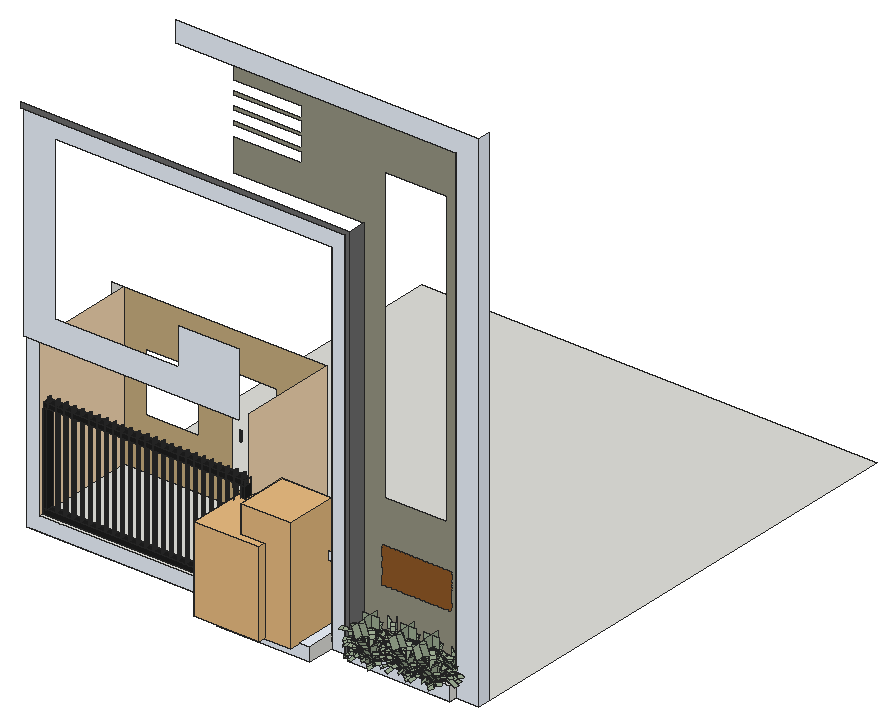
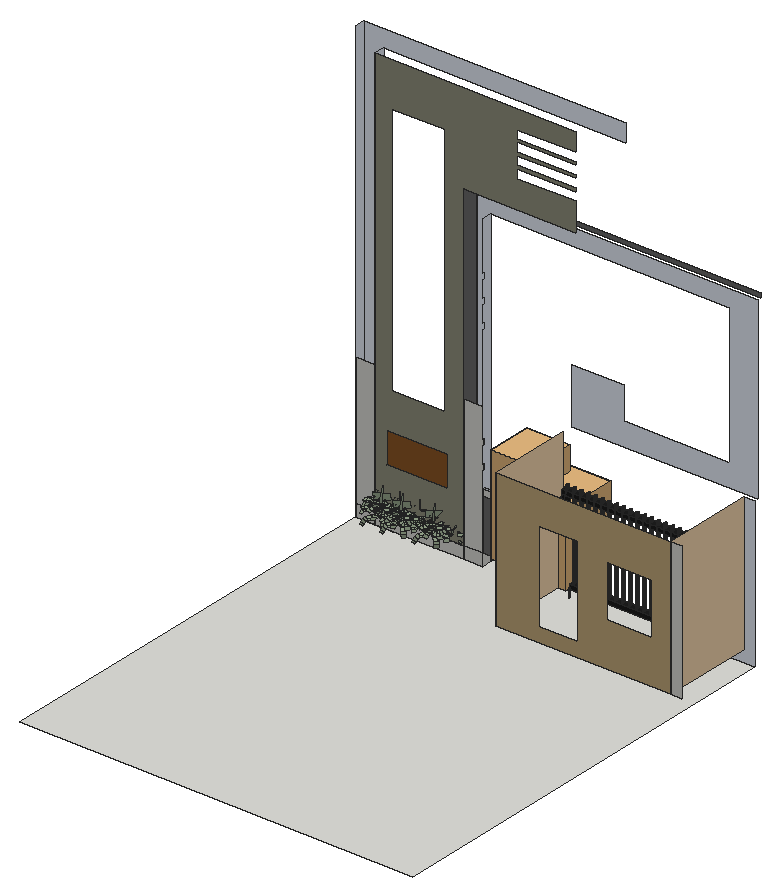
# SketchUp Ruby script. Lengths in inches.
U = 1.inch
M = Sketchup.active_model
def pt(a) = Geom::Point3d.new(a.map { |v| v * U })
def face(e, loops, mat)
  f = e.add_face(loops[0].map { |a| pt(a) })
  loops[1..].each { |l| e.add_face(l.map { |a| pt(a) }).erase! }
  f.material = f.back_material = mat if mat
  f
end
# faces: each face lists its corners as indices into pts; further lists are holes
def faces(e, pts, list, mat = nil) = list.each { |f| face(e, (f[0].is_a?(Array) ? f : [f]).map { |l| l.map { |i| pts[i] } }, mat) }
# xy, xz, yz: faces in a plane at the given z, y or x. An outline is a flat list of corners, or four numbers for a rectangle; further outlines are holes
def ring(l) = l.size == 4 ? [[l[0], l[1]], [l[2], l[1]], [l[2], l[3]], [l[0], l[3]]] : l.each_slice(2).to_a
def flat(e, list, mat, &to3) = list.each { |f| face(e, (f[0].is_a?(Array) ? f : [f]).map { |l| ring(l).map { |u, v| to3.(u, v) } }, mat) }
def xy(e, z, list, mat = nil) = flat(e, list, mat) { |x, y| [x, y, z] }
def xz(e, y, list, mat = nil) = flat(e, list, mat) { |x, z| [x, y, z] }
def yz(e, x, list, mat = nil) = flat(e, list, mat) { |y, z| [x, y, z] }
def lines(e, pts, list) = list.each { |a, b| e.add_line(pt(pts[a]), pt(pts[b])) }
# prism: a flat outline (further loops are holes) pulled along v
def prism(e, loops, v, mat = nil)
  f = face(e, loops, mat); d = Geom::Vector3d.new(v.map { |x| x * U })
  f.pushpull(f.normal.samedirection?(d) ? d.length : -d.length)
end
def box(e, o, s, mat = nil) = prism(e, [[o, [o[0] + s[0], o[1], o[2]], [o[0] + s[0], o[1] + s[1], o[2]], [o[0], o[1] + s[1], o[2]]]], [0, 0, s[2]], mat)
def at(x, y, z, deg = 0) = Geom::Transformation.translation(pt([x, y, z])) * Geom::Transformation.rotation(ORIGIN, Z_AXIS, deg.degrees)
def axes(o, x, y, z) = Geom::Transformation.new([*x, 0, *y, 0, *z, 0, *pt(o).to_a, 1])
def part(name) = M.definitions.add(name)
# library, detail: a bought-in or finely detailed component or shape, given as its bounding box
def library(name, o, s) = part(name).tap { |d| box(d.entities, o, s) }
def detail(e, o, s) = box(e.add_group.entities, o, s)
def put(e, d, t, mat = nil) = e.add_instance(d, t).tap { |i| i.material = mat if mat }
def group(e, t, mat = nil) = e.add_group.tap { |g| g.transformation = t; g.material = mat if mat }.entities
root = M.entities
M.materials.add("Generic").color = [111, 111, 111]
M.materials.add("Generic\#2").color = [253, 222, 182]
M.materials.add("Generic\#3").color = [151, 150, 132]
M.materials.add("Generic\#4").color = [238, 245, 255]
M.materials.add("Material \#1").color = [140, 140, 140]
M.materials.add("[Color M08]").color = [30, 30, 30]
M.materials.add("[Roofing Slate Tan]").color = [200, 175, 128]
M.materials.add("[Wood Floor Parquet]").color = [145, 89, 39]
M.materials.add("hymenocallis littoralis").color = [156, 172, 146]
c1 = library("Plant+2 (1)",[-9.13,-9.52,0],[51.76,51.77,66.88])
c2 = library("Plant",[-27.84,-31.84,-1.26],[68.28,70.82,154.38])
c3 = part("Group\#856")
xy(c3.entities,7.38,[[0,0,5.5,15.91]],"hymenocallis littoralis")
p = [[5.5,28.78,0],[5.5,26.79,3.44],[0,26.79,3.44],[0,28.78,0],[0,23.75,6],[5.5,23.75,6],
  [0,15.91,7.38],[5.5,15.91,7.38]]
faces(c3.entities,p,[[0,1,2,3],[4,2,1,5],[6,4,5,7]],"hymenocallis littoralis")
c4 = part("Group\#854")
xy(c4.entities,7.38,[[0,0,5.5,15.91],[0,15.91,5.5,23.87]],"hymenocallis littoralis")
p = [[5.5,31.07,4.3],[5.5,27.74,6.47],[0,27.74,6.47],[0,31.07,4.3],[0,23.87,7.38],[5.5,23.87,7.38]]
faces(c4.entities,p,[[0,1,2,3],[4,2,1,5]],"hymenocallis littoralis")
c5 = part("Group\#857")
xy(c5.entities,7.38,[[0,0,5.6,15.91]],"hymenocallis littoralis")
p = [[5.6,28.78,0],[5.6,26.79,3.44],[0,26.79,3.44],[0,28.78,0],[0,23.75,6],[5.6,23.75,6],
  [0,15.91,7.38],[5.6,15.91,7.38]]
faces(c5.entities,p,[[0,1,2,3],[4,2,1,5],[6,4,5,7]],"hymenocallis littoralis")
c6 = part("Group\#855")
put(c6.entities,c4,axes([6.09,8.57,-0.52],[0.446,0.85617,0.26089],[-0.18444,-0.19731,0.96283],[0.87582,-0.47754,0.0699]))
put(c6.entities,c4,axes([6.29,7.28,-1.71],[0.37058,0.92707,-0.05667],[-0.32382,0.19004,0.99128],[0.87712,-0.32925,0.34964]))
put(c6.entities,c4,axes([11.04,16.14,-0.7],[1,0,0],[0,0.16628,1.02662],[0,-1.18456,0.19186]))
c7 = part("Group\#860")
put(c7.entities,c3,axes([24.57,32.05,-1.76],[0.9552,-0.22102,-0.19681],[0.4036,0.95545,0.88585],[-0.00568,-0.67859,0.7345]))
put(c7.entities,c3,axes([23.95,29.24,-2.4],[0,1,0],[-0.76041,0,0.64945],[0.64945,0,0.76041]))
put(c7.entities,c3,axes([24.22,24.72,-0.48],[-0.70711,0.70711,0],[-0.32757,-0.32757,0.80237],[0.61237,0.61237,0.5]))
put(c7.entities,c4,axes([20.66,37.22,-0.63],[1.12361,0.03262,0.39091],[-0.43499,0.29739,0.78777],[0.09852,-1.27434,0.37535]))
put(c7.entities,c3,axes([28.75,24.45,-2.4],[-1,0,0],[0,-0.76041,0.64945],[0,0.64945,0.76041]))
put(c7.entities,c5,axes([30.4,30.98,-3.7],[0.65676,-0.72002,0.22414],[0.55667,0.66341,0.5],[-0.50871,-0.20361,0.83652]))
put(c7.entities,c5,axes([32.41,29.61,-3.7],[0.04029,-0.97372,0.22414],[0.85287,0.15038,0.5],[-0.52057,0.17102,0.83652]))
put(c7.entities,c3,axes([31.89,25.85,-1.76],[-0.92056,0.33739,-0.19681],[-0.5186,-0.89824,0.88585],[0.08952,0.67268,0.7345]))
put(c7.entities,c3,axes([25.55,34.78,-0.48],[0.86603,0.5,0],[-0.25,0.43301,0.86603],[0.43301,-0.75,0.5]))
put(c7.entities,c5,axes([20.4,16.9375,-8.07],[-0.70711,0.70711,0],[-0.35754,-0.35754,0.65422],[1.3987,1.3987,1.52882]))
put(c7.entities,c3,axes([32.86,34.14,-0.48],[0.76604,-0.64279,0],[0.32139,0.38302,0.86603],[-0.55667,-0.66341,0.5]))
put(c7.entities,c3,axes([27.15,34.7,-0.1],[0.82472,-0.17528,-0.53769],[0.53769,0.53769,0.64945],[0.17528,-0.82472,0.53769]))
put(c7.entities,c3,axes([33.58,28.77,-2.4],[0,-1,0],[0.76041,0,0.64945],[-0.64945,0,0.76041]))
put(c7.entities,c3,axes([26.43,23.87,-2.81],[-0.75126,0.04415,0.65853],[0.53769,-0.53769,0.64945],[0.38276,0.84199,0.3802]))
put(c7.entities,c3,axes([28.78,23.98,-2.4],[-1,0,0],[0,-0.76041,0.64945],[0,0.64945,0.76041]))
put(c7.entities,c3,axes([25.39,25.38,-2.4],[-0.70711,0.70711,0],[-0.53769,-0.53769,0.64945],[0.45923,0.45923,0.76041]))
put(c7.entities,c3,axes([27.32,21.63,-0.1],[-0.45923,0.70711,-0.53769],[-0.76041,0,0.64945],[0.45923,0.70711,0.53769]))
put(c7.entities,c3,axes([25.17,27.625,-1.76],[0.56416,0.80187,-0.19681],[-0.66673,0.66673,0.80532],[0.62659,-0.26057,0.7345]))
put(c7.entities,c5,axes([27.59,27.04,-3.96],[-0.8993,-0.06127,0.43301],[0.2962,-0.8138,0.5],[0.32175,0.57791,0.75]))
put(c7.entities,c5,axes([26.98,24.5,-3.18],[-0.5,0.86603,0],[-0.75,-0.43301,0.5],[0.43301,0.25,0.86603]))
put(c7.entities,c5,axes([24.55,27.74,-3.7],[0.29517,0.92878,0.22414],[-0.85287,0.15038,0.5],[0.43068,-0.33875,0.83652]))
put(c7.entities,c5,axes([24.26,29.8,-3.18],[0.76604,0.64279,0],[-0.47317,0.5639,0.425],[0.32139,-0.38302,0.86603]))
put(c7.entities,c5,axes([25.98,32.46,-3.18],[1,0,0],[0,0.86603,0.5],[0,-0.5,0.86603]))
put(c7.entities,c3,axes([28.78,33.57,-2.4],[1,0,0],[0,0.76041,0.64945],[0,-0.64945,0.76041]))
put(c7.entities,c6,at(14.99,21.38,2.5))
put(c7.entities,c4,axes([34.63,26.34,-1.46],[-0.70089,-0.70877,0.07994],[0.4756,-0.38088,0.79293],[-0.53156,0.59378,0.60405]))
put(c7.entities,c4,axes([28.14,16.92,1.8125],[-1.19719,0.6912,0],[-0.09607,-0.16641,0.94244],[0.68444,1.18549,0.17613]))
put(c7.entities,c4,axes([31.5625,35.84,0.97],[0.66765,-1.1564,0.35779],[0.04445,0.30732,0.91033],[-1.20828,-0.64496,0.17012]))
put(c7.entities,c4,axes([38.94,22.51,0.89],[-0.97932,-0.67164,-0.05202],[0.27787,-0.41401,0.90999],[-0.85985,0.93577,0.32097]))
put(c7.entities,c4,axes([38.44,21.09,1.98],[-1.02864,-0.54856,0.2395],[0.33481,0.06999,0.88388],[-0.77261,1.08328,0.06417]))
put(c7.entities,c5,axes([35.02,30.51,-1.3],[-0.17365,-0.98481,0],[0.60224,-0.10619,0.79122],[-0.7792,0.13739,0.61153]))
put(c7.entities,c5,axes([29.41,22.33,-1.3],[-0.93969,0.34202,0],[-0.20915,-0.57465,0.79122],[0.27061,0.74351,0.61153]))
put(c7.entities,c4,axes([19.64,36,-1.62],[1.18194,0.09546,0.08234],[-0.14377,0.68823,0.76313],[0.21457,-1.1326,0.62386]))
put(c7.entities,c5,axes([24.25,24.14,-1.3],[-0.34202,0.93969,0],[-0.57465,-0.20915,0.79122],[0.74351,0.27061,0.61153]))
put(c7.entities,c5,axes([25.98,34.61,-1.3],[1,0,0],[0,0.61153,0.79122],[0,-0.79122,0.61153]))
put(c7.entities,c5,axes([31.16,34.41,-1.64],[0.56518,-0.80224,-0.19234],[0.73413,0.34233,0.72935],[-0.47639,-0.50772,0.71782]))
put(c7.entities,c5,axes([40.52,26.84,-5.82],[-0.42262,-0.90631,0],[0.48019,-0.22391,0.68552],[-1.43418,0.66877,1.22305]))
put(c7.entities,c3,axes([29.86,38.42,-1.01],[0.89064,-0.37013,0.26413],[-0.03924,0.63286,1.01918],[-0.45353,-0.76487,0.45748]))
put(c7.entities,c3,axes([29.34,22.4,-0.48],[-0.99619,-0.08716,0],[0.04358,-0.4981,0.86603],[-0.07548,0.86273,0.5]))
c8 = part("Group\#858")
xz(c8.entities,10.07,[[9.07,0,10.07,31.01],[0,31.01,0,45.12,20.13,45.12,20.13,31.01,10.07,31.01,10.07,32.58,9.07,32.58,9.07,31.01]],"hymenocallis littoralis")
yz(c8.entities,10.07,[[0,31.01,20.13,45.12]],"hymenocallis littoralis")
p = [[9.57,9.2,0],[10.07,10.07,0],[10.07,10.07,31.01],[10.07,10.07,32.58],[9.57,9.2,32.58]]
faces(c8.entities,p,[[0,1,2,3,4]],"hymenocallis littoralis")
c9 = part("cây lá nắng")
put(c9.entities,c7,axes([49.26,-2.75,0],[0.63109,0.63109,0],[-0.63109,0.63109,0],[0,0,0.935]))
g1 = group(c9.entities,at(26.6,-8.68,0))
put(g1,c3,axes([-4.72,35.73,-1.65],[0.74231,0.46334,-0.18402],[-0.34827,0.85768,0.82827],[0.42467,-0.43184,0.68675]))
put(g1,c3,axes([-3.34,33.57,-2.24],[-0.63109,0.63109,0],[-0.47989,-0.47989,0.60723],[0.40986,0.40986,0.71098]))
put(g1,c3,axes([-0.3125,30.89,-0.45],[-0.8925,0,0],[0,-0.41345,0.75022],[0,0.77293,0.4675]))
put(g1,c4,axes([-10.79,39.66,-0.59],[0.68852,0.72969,0.3655],[-0.4622,-0.08684,0.73657],[0.86641,-0.74205,0.35095]))
put(g1,c3,axes([2.71,33.57,-2.24],[-0.63109,-0.63109,0],[0.47989,-0.47989,0.60723],[-0.40986,0.40986,0.71098]))
put(g1,c5,axes([-0.37,38.74,-3.46],[0.86887,-0.03992,0.20957],[-0.06737,0.76999,0.4675],[-0.19255,-0.44954,0.78214]))
put(g1,c5,axes([1.76,39.14,-3.46],[0.63993,-0.58908,0.20957],[0.44333,0.63315,0.4675],[-0.43646,-0.2206,0.78214]))
put(g1,c3,axes([3.81,36.4375,-1.65],[-0.79389,-0.36803,-0.18402],[0.23959,-0.89415,0.82827],[-0.36803,0.48102,0.68675]))
put(g1,c3,axes([-5.83,38.07,-0.45],[0.231,0.86209,0],[-0.43104,0.1155,0.80973],[0.74659,-0.20005,0.4675]))
put(g1,c5,axes([2.18,23.5625,-7.55],[-0.8925,0,0],[0,-0.45128,0.6117],[0,1.76542,1.42944]))
put(g1,c3,axes([-0.8125,42.28,-0.45],[0.8891,0.07779,0],[-0.03889,0.44455,0.80973],[0.06737,-0.76999,0.4675]))
put(g1,c3,axes([-4.76,39.03,-0.09],[0.63109,0.40986,-0.50274],[0,0.67866,0.60723],[0.63109,-0.40986,0.50274]))
put(g1,c3,axes([3.03,39.35,-2.24],[0.63109,-0.63109,0],[0.47989,0.47989,0.60723],[-0.40986,-0.40986,0.71098]))
put(g1,c3,axes([1.61,31.74,-2.625],[-0.50198,-0.44625,0.61573],[0.67866,0,0.60723],[-0.28982,0.77293,0.35549]))
put(g1,c3,axes([3.03,33.3,-2.24],[-0.63109,-0.63109,0],[0.47989,-0.47989,0.60723],[-0.40986,0.40986,0.71098]))
put(g1,c3,axes([0.01,32.04,-2.24],[-0.8925,0,0],[0,-0.67866,0.60723],[0,0.57963,0.71098]))
put(g1,c3,axes([3.59,30.89,-0.09],[-0.73607,0.15643,-0.50274],[-0.47989,-0.47989,0.60723],[-0.15643,0.73607,0.50274]))
put(g1,c3,axes([-1.55,33.32,-1.65],[-0.15002,0.86209,-0.18402],[-0.84154,0,0.75297],[0.55988,0.231,0.68675]))
put(g1,c5,axes([0.35,34.48,-3.71],[-0.52887,-0.60621,0.40487],[0.70051,-0.32665,0.4675],[-0.16166,0.56777,0.70125]))
put(g1,c5,axes([2.61,39.13,-1.74],[-0.86209,0.231,0],[-0.23031,-0.85954,0.15531],[0.03162,0.11799,0.91645]))
put(g1,c5,axes([-2.02,33,-3.46],[-0.39986,0.77243,0.20957],[-0.63315,-0.44333,0.4675],[0.48558,0.05802,0.78214]))
put(g1,c5,axes([-3.49,34.12,-2.97],[0.07779,0.8891,0],[-0.65449,0.05726,0.39737],[0.44455,-0.03889,0.80973]))
put(g1,c5,axes([-4.09,36.88,-2.97],[0.63109,0.63109,0],[-0.54654,0.54654,0.4675],[0.31555,-0.31555,0.80973]))
put(g1,c3,axes([-3.02,39.35,-2.24],[0.63109,0.63109,0],[-0.47989,0.47989,0.60723],[0.40986,-0.40986,0.71098]))
put(g1,c6,axes([-4.03,22.95,2.33],[0.63109,0.63109,0],[-0.63109,0.63109,0],[0,0,0.935]))
put(g1,c4,axes([5.24,38.48,-1.37],[0.00497,-0.88963,0.07474],[0.54052,0.05978,0.74139],[-0.71019,0.03927,0.56479]))
put(g1,c4,axes([7.08,28.4375,1.7],[-1.19175,-0.31933,0],[0.04439,-0.16565,0.88118],[-0.31621,1.1801,0.16468]))
put(g1,c4,axes([-2.7,42.54,0.91],[1.15114,-0.30845,0.33454],[-0.1659,0.22199,0.85115],[-0.3555,-1.16957,0.15907]))
put(g1,c4,axes([10.37,38.78,0.83],[-0.19417,-1.04191,-0.04864],[0.43664,-0.08592,0.85084],[-1.1332,0.04791,0.30011]))
put(g1,c4,axes([10.95,37.5625,1.85],[-0.30298,-0.99536,0.22393],[0.16713,0.25547,0.82643],[-1.17124,0.19607,0.06]))
put(g1,c5,axes([2.84,41.36,-1.22],[0.51192,-0.73109,0],[0.44708,0.31305,0.73979],[-0.57846,-0.40504,0.57178]))
put(g1,c5,axes([4.47,32.65,-1.22],[-0.80888,-0.37719,0],[0.23066,-0.49465,0.73979],[-0.29844,0.64,0.57178]))
put(g1,c4,axes([-10.32,35.12,-1.51],[0.68567,0.80616,0.07699],[-0.52507,0.3436,0.71352],[0.85019,-0.57936,0.58331]))
put(g1,c5,axes([0.07,30.54,-1.22],[-0.80888,0.37719,0],[-0.23066,-0.49465,0.73979],[0.29844,0.64,0.57178]))
put(g1,c5,axes([-5.45,38.24,-1.22],[0.63109,0.63109,0],[-0.38593,0.38593,0.73979],[0.49934,-0.49934,0.57178]))
put(g1,c5,axes([-2.05,41.38,-1.53],[0.86296,-0.14961,-0.17984],[0.24726,0.67935,0.68194],[0.01977,-0.62107,0.67116]))
put(g1,c5,axes([8.63,42.51,-5.4375],[0.30525,-0.83868,0],[0.44435,0.16173,0.64096],[-1.32716,-0.48305,1.14356]))
put(g1,c3,axes([-5.4,43.09,-0.94],[0.79566,0.32849,0.24696],[-0.42416,0.37462,0.95293],[0.19648,-0.76892,0.42774]))
put(g1,c3,axes([4.38,32.65,-0.45],[-0.57369,-0.68369,0],[0.34185,-0.28684,0.80973],[-0.5921,0.49683,0.4675]))
put(g1,c5,axes([-2,33.84,-0.15],[-0.24601,0.85793,0],[-0.85539,-0.24528,0.15531],[0.11742,0.03367,0.91645]))
put(g1,c5,axes([0.17,30.83,-4.47],[-0.24601,0.85793,0],[-0.85539,-0.24528,0.15531],[0.11742,0.03367,0.91645]))
put(g1,c5,axes([-1.97,32.18,-4.47],[0.58524,0.67383,0],[-0.67184,0.58351,0.15531],[0.09222,-0.0801,0.91645]))
put(g1,c5,axes([-2,34.71,-4.47],[0.88392,-0.12346,0],[0.12309,0.88131,0.15531],[-0.0169,-0.12098,0.91645]))
put(g1,c5,axes([0.11,36.12,-4.47],[0.37822,-0.8084,0],[0.80601,0.37711,0.15531],[-0.11064,-0.05177,0.91645]))
put(c9.entities,c8,axes([29.71,14.29,6.94],[0.425,0.73612,0],[-0.6771,0.39092,-0.33349],[-0.26859,0.15507,0.72712]))
put(c9.entities,c8,axes([42.0625,26.12,6.94],[0.85,0,0],[0,0.78185,-0.33349],[0,0.33349,0.78185]))
put(c9.entities,c7,axes([7.3125,23.0625,0],[0.8925,0,0],[0,0.8925,0],[0,0,0.935]))
put(c9.entities,c8,axes([24.4375,40.23,2.05],[0.85,0,0],[0,0.85,0],[0,0,0.85]))
c10 = part("Planting+101")
put(c10.entities,c9,axes([21.34,32.96,-4.59],[0,-0.71,0],[-0.71,0,0],[0,0,0.71]))
c11 = part("Group\#428")
prism(c11.entities,[[[0,1.97,0],[0,1.97,1.18],[0,0,1.18],[0,0,0]],[[0,1.92,1.13],[0,1.92,0.05],[0,0.05,0.05],[0,0.05,1.13]]],[98.43,0,0])
c12 = part("Group\#430")
xy(c12.entities,0,[[0.3,0,0.22,0.01,0.15,0.04,0.09,0.09,0.04,0.15,0.01,0.22,0,0.3,0.3,0.3],[0.3,0,0.3,0.3,0.59,0.3,0.58,0.22,0.55,0.15,0.5,0.09,0.44,0.04,0.37,0.01],[0,0.3,0.01,0.37,0.04,0.44,0.09,0.5,0.15,0.55,0.22,0.58,0.3,0.59,0.3,0.3],[0.3,0.3,0.3,0.59,0.37,0.58,0.44,0.55,0.5,0.5,0.55,0.44,0.58,0.37,0.59,0.3]])
xy(c12.entities,39.37,[[0.3,0,0.37,0.01,0.44,0.04,0.5,0.09,0.55,0.15,0.58,0.22,0.59,0.3,0.58,0.37,0.55,0.44,0.5,0.5,0.44,0.55,0.37,0.58,0.3,0.59,0.22,0.58,0.15,0.55,0.09,0.5,0.04,0.44,0.01,0.37,0,0.3,0.01,0.22,0.04,0.15,0.09,0.09,0.15,0.04,0.22,0.01]])
p = [[0.09,0.09,0],[0.15,0.04,0],[0.15,0.04,39.37],[0.09,0.09,39.37],[0.22,0.01,0],[0.22,0.01,39.37],
  [0.3,0,0],[0.3,0,39.37],[0.37,0.01,0],[0.37,0.01,39.37],[0.44,0.04,0],[0.44,0.04,39.37],
  [0.5,0.09,0],[0.5,0.09,39.37],[0.01,0.22,0],[0.04,0.15,0],[0.04,0.15,39.37],[0.01,0.22,39.37],
  [0.55,0.15,0],[0.55,0.15,39.37],[0.58,0.22,0],[0.58,0.22,39.37],[0,0.3,0],[0,0.3,39.37],
  [0.59,0.3,0],[0.59,0.3,39.37],[0.01,0.37,0],[0.01,0.37,39.37],[0.58,0.37,0],[0.58,0.37,39.37],
  [0.09,0.5,0],[0.04,0.44,0],[0.04,0.44,39.37],[0.09,0.5,39.37],[0.55,0.44,0],[0.5,0.5,0],
  [0.5,0.5,39.37],[0.55,0.44,39.37],[0.15,0.55,0],[0.15,0.55,39.37],[0.44,0.55,0],[0.44,0.55,39.37],
  [0.22,0.58,0],[0.22,0.58,39.37],[0.3,0.59,0],[0.3,0.59,39.37],[0.37,0.58,0],[0.37,0.58,39.37]]
faces(c12.entities,p,[[0,1,2,3],[1,4,5,2],[4,6,7,5],[6,8,9,7],[8,10,11,9],[10,12,13,11],[14,15,16,17],[15,0,3,16],
  [12,18,19,13],[18,20,21,19],[22,14,17,23],[20,24,25,21],[26,22,23,27],[24,28,29,25],[30,31,32,33],[31,26,27,32],
  [34,35,36,37],[28,34,37,29],[38,30,33,39],[35,40,41,36],[42,38,39,43],[44,42,43,45],[46,44,45,47],[40,46,47,41]])
c13 = part("Group\#429")
prism(c13.entities,[[[0.01,0.22,35.83],[0,0.3,35.83],[0.01,0.37,35.83],[0.04,0.44,35.83],[0.09,0.5,35.83],[0.15,0.55,35.83],[0.22,0.58,35.83],[0.3,0.59,35.83],[0.37,0.58,35.83],[0.44,0.55,35.83],[0.5,0.5,35.83],[0.55,0.44,35.83],[0.58,0.37,35.83],[0.59,0.3,35.83],[0.58,0.22,35.83],[0.55,0.15,35.83],[0.5,0.09,35.83],[0.44,0.04,35.83],[0.37,0.01,35.83],[0.3,0,35.83],[0.22,0.01,35.83],[0.15,0.04,35.83],[0.09,0.09,35.83],[0.04,0.15,35.83]]],[0,0,3.54])
c14 = part("Metal railing panel")
g2 = group(c14.entities,at(0,0,0))
put(g2,c11,axes([0,0,39.76],[1,0,0],[0,0,-1],[0,1,0]),"[Color M08]")
put(g2,c11,axes([0,0,1.97],[1,0,0],[0,0,-1],[0,1,0]),"[Color M08]")
put(g2,c11,axes([98.43,0,37.8],[0,0,-0.364],[-1,0,0],[0,1,0]),"[Color M08]")
put(g2,c11,axes([1.97,0,37.8],[0,0,-0.364],[-1,0,0],[0,1,0]),"[Color M08]")
g3 = group(c14.entities,at(1.67,0.3,1.97))
put(g3,c12,at(78.74,0,0),"[Color M08]")
put(g3,c12,at(90.55,0,0),"[Color M08]")
put(g3,c12,at(82.68,0,0),"[Color M08]")
put(g3,c12,at(86.61,0,0),"[Color M08]")
put(g3,c12,at(66.93,0,0),"[Color M08]")
put(g3,c12,at(11.8125,0,0),"[Color M08]")
put(g3,c12,at(15.75,0,0),"[Color M08]")
put(g3,c12,at(47.24,0,0),"[Color M08]")
put(g3,c12,at(59.06,0,0),"[Color M08]")
put(g3,c13,at(0,0,0),"[Color M08]")
put(g3,c12,at(39.37,0,0),"[Color M08]")
put(g3,c12,at(62.99,0,0),"[Color M08]")
put(g3,c12,at(55.12,0,0),"[Color M08]")
put(g3,c12,at(19.69,0,0),"[Color M08]")
put(g3,c12,at(35.43,0,0),"[Color M08]")
put(g3,c12,at(7.875,0,0),"[Color M08]")
put(g3,c12,at(23.62,0,0),"[Color M08]")
put(g3,c12,at(31.5,0,0),"[Color M08]")
put(g3,c12,at(43.31,0,0),"[Color M08]")
put(g3,c12,at(27.56,0,0),"[Color M08]")
put(g3,c12,at(3.9375,0,0),"[Color M08]")
put(g3,c12,at(51.18,0,0),"[Color M08]")
put(g3,c12,at(70.87,0,0),"[Color M08]")
put(g3,c12,at(74.8,0,0),"[Color M08]")
put(g3,c13,at(94.49,0,0),"[Color M08]")
xy(root,-11.1875,[[169.979,6.341,169.979,30.841,0,30.841,0,421.591,360,421.591,360,37.591,243.692,37.591,243.692,6.341],[260.974,21.778,342.12,37.591],[257.286,24.153,257.286,27.716,243.692,27.716,243.692,37.591,260.974,37.591,260.974,24.153],[342.12,27.716,360,37.591]])
xy(root,-8.25,[[263.421,24.225,339.673,35.144]])
xy(root,0,[[[260.974,21.778,342.12,37.591],[263.421,24.225,339.673,35.144]],[9.75,30.841,169.979,114.716]])
xy(root,0,[[169.979,6.341,243.692,37.591]],"Generic\#4")
xy(root,46.439,[[169.979,34.653,243.692,37.591]])
xz(root,6.341,[[169.979,-11.1875,243.692,0]],"Generic\#4")
xz(root,21.778,[[260.974,-11.1875,342.12,0]],"Generic\#4")
xz(root,24.153,[[257.286,-11.1875,260.974,-11.1875,260.974,292.75,0,292.75,0,288.8125,257.286,288.8125]],"Generic")
xz(root,24.225,[[263.421,-8.25,339.673,0]])
xz(root,27.716,[[243.692,-11.1875,257.286,-11.1875,257.286,288.8125,0,288.8125,0,125.3125,169.979,125.3125,169.979,175.6875,122.632,175.6875,122.632,146.375,24.805,146.375,24.805,273.875,243.692,273.875],[342.12,-11.1875,360,-11.1875,360,391.636,120.099,391.636,120.099,375.448,342.12,375.448]],"Generic\#4")
xz(root,30.841,[[0,-11.1875,169.979,-11.1875,169.979,0,9.75,0,9.75,125.3125,0,125.3125]],"Generic\#4")
xz(root,34.653,[[169.979,46.439,243.692,52.376]],"Generic\#4")
xz(root,35.144,[[263.421,-8.25,339.673,0]])
xz(root,37.591,[[243.692,-11.1875,260.974,0],[260.974,-11.1875,342.12,0],[342.12,-11.1875,360,0],[243.692,0,260.974,120],[342.12,0,360,120],
  [169.979,46.439,243.692,52.376]])
xz(root,37.591,[[169.979,0,243.692,46.439]],"Generic")
xz(root,37.591,[[[260.974,0,342.12,0,342.12,375.448,158.474,375.448,158.474,358.525,211.974,358.525,211.974,350.4,158.474,350.4,158.474,347.9,211.974,347.9,211.974,339.775,158.474,339.775,158.474,337.15,211.974,337.15,211.974,329.025,158.474,329.025,158.474,326.4,211.974,326.4,211.974,318.275,158.474,318.275,158.474,292.75,260.974,292.75],[278.093,103.872,326.77,335.362],[275.776,41.247,331.151,70.06]]],"Generic\#3")
xz(root,37.591,[[275.776,41.247,331.151,70.06]],"[Wood Floor Parquet]")
xz(root,114.716,[[0,0,9.75,125.3125]])
xz(root,114.716,[[[9.75,0,169.979,125.3125],[95.002,12.899,130.44,95.774],[27.056,40.409,68.556,87.784]]],"[Roofing Slate Tan]")
xz(root,115.852,[[101.393,47.076,101.29,47.087,101.393,47.087],[101.393,47.076,101.393,47.087,101.494,47.098],[101.393,47.076,101.494,47.098,101.496,47.087],[101.29,47.087,101.193,47.118,101.291,47.098],[101.29,47.087,101.291,47.098,101.393,47.087],
  [101.496,47.087,101.494,47.098,101.589,47.129],[101.496,47.087,101.589,47.129,101.593,47.118],[101.291,47.098,101.193,47.118,101.196,47.129],[101.193,47.118,101.103,47.168,101.196,47.129],[101.593,47.118,101.589,47.129,101.677,47.178],
  [101.593,47.118,101.677,47.178,101.682,47.168],[101.196,47.129,101.103,47.168,101.108,47.178],[101.103,47.168,101.023,47.235,101.108,47.178],[101.682,47.168,101.677,47.178,101.756,47.244],[101.682,47.168,101.756,47.244,101.762,47.235],
  [101.108,47.178,101.023,47.235,101.03,47.244],[101.023,47.235,100.954,47.317,101.03,47.244],[101.762,47.235,101.756,47.244,101.824,47.324],[101.762,47.235,101.824,47.324,101.832,47.317],[101.03,47.244,100.954,47.317,100.961,47.324],
  [101.393,47.257,101.359,47.26,101.393,47.268],[101.393,47.257,101.393,47.268,101.425,47.272],[101.393,47.257,101.425,47.272,101.427,47.26],[101.359,47.26,101.326,47.271,101.36,47.272],[101.359,47.26,101.36,47.272,101.393,47.268],
  [101.427,47.26,101.425,47.272,101.456,47.282],[101.427,47.26,101.456,47.282,101.459,47.271],[101.326,47.271,101.297,47.288,101.33,47.282],[101.326,47.271,101.33,47.282,101.36,47.272],[101.459,47.271,101.456,47.282,101.484,47.298],
  [101.459,47.271,101.484,47.298,101.489,47.288],[101.33,47.282,101.297,47.288,101.302,47.298],[101.297,47.288,101.27,47.31,101.302,47.298],[101.489,47.288,101.484,47.298,101.509,47.319],[101.489,47.288,101.509,47.319,101.516,47.31],
  [101.302,47.298,101.27,47.31,101.276,47.319],[101.27,47.31,101.247,47.337,101.276,47.319],[101.516,47.31,101.509,47.319,101.531,47.344],[101.516,47.31,101.531,47.344,101.539,47.337],[101.832,47.317,101.824,47.324,101.88,47.417],
  [101.832,47.317,101.88,47.417,101.888,47.411],[101.276,47.319,101.247,47.337,101.255,47.344],[101.247,47.337,101.228,47.368,101.255,47.344],[101.539,47.337,101.531,47.344,101.549,47.374],[101.539,47.337,101.549,47.374,101.557,47.368],
  [101.255,47.344,101.228,47.368,101.237,47.374],[101.557,47.368,101.549,47.374,101.562,47.407],[101.557,47.368,101.562,47.407,101.571,47.403],[101.571,47.403,101.562,47.407,101.571,47.444],[101.571,47.403,101.571,47.444,101.58,47.442],
  [100.9,47.405,100.855,47.517,100.909,47.411],[100.909,47.411,100.855,47.517,100.864,47.521],[101.58,47.442,101.571,47.444,101.574,47.482],[101.58,47.442,101.574,47.482,101.583,47.482],[101.215,47.444,101.202,47.478,101.212,47.478],
  [101.202,47.478,101.205,47.522,101.212,47.478],[101.212,47.478,101.205,47.522,101.215,47.52],[101.574,47.482,101.571,47.52,101.583,47.482],[101.583,47.482,101.571,47.52,101.58,47.522],[100.855,47.517,100.828,47.631,100.864,47.521],
  [101.931,47.517,101.921,47.521,101.948,47.633],[101.931,47.517,101.948,47.633,101.957,47.631],[101.215,47.52,101.205,47.522,101.214,47.56],[101.215,47.52,101.214,47.56,101.223,47.556],[101.571,47.52,101.562,47.556,101.58,47.522],
  [100.864,47.521,100.828,47.631,100.838,47.633],[101.58,47.522,101.562,47.556,101.571,47.56],[101.223,47.556,101.214,47.56,101.228,47.595],[101.223,47.556,101.228,47.595,101.237,47.59],[101.562,47.556,101.549,47.59,101.571,47.56],
  [101.571,47.56,101.549,47.59,101.557,47.595],[101.237,47.59,101.228,47.595,101.247,47.627],[101.237,47.59,101.247,47.627,101.255,47.619],[101.549,47.59,101.531,47.619,101.557,47.595],[101.557,47.595,101.531,47.619,101.539,47.627],
  [101.255,47.619,101.247,47.627,101.27,47.654],[101.255,47.619,101.27,47.654,101.276,47.645],[101.531,47.619,101.509,47.645,101.539,47.627],[101.539,47.627,101.509,47.645,101.516,47.654],[100.828,47.631,100.819,47.757,100.838,47.633],
  [101.957,47.631,101.948,47.633,101.957,47.758],[101.957,47.631,101.957,47.758,101.967,47.757],[100.838,47.633,100.819,47.757,100.828,47.758],[101.276,47.645,101.27,47.654,101.297,47.676],[101.509,47.645,101.484,47.666,101.516,47.654],
  [101.516,47.654,101.484,47.666,101.489,47.676],[101.302,47.666,101.297,47.676,101.326,47.693],[101.302,47.666,101.326,47.693,101.33,47.682],[101.484,47.666,101.456,47.682,101.489,47.676],[101.489,47.676,101.456,47.682,101.459,47.693],
  [101.33,47.682,101.326,47.693,101.359,47.703],[101.33,47.682,101.359,47.703,101.36,47.692],[101.456,47.682,101.425,47.692,101.459,47.693],[101.36,47.692,101.359,47.703,101.393,47.707],[101.36,47.692,101.393,47.707,101.393,47.695],
  [101.425,47.692,101.393,47.695,101.427,47.703],[101.425,47.692,101.427,47.703,101.459,47.693],[101.393,47.695,101.393,47.707,101.427,47.703],[100.819,47.757,100.819,55.494,100.828,47.758],[101.967,47.757,101.957,47.758,101.957,53.826],
  [101.967,47.757,101.957,53.826,101.957,55.493],[101.967,47.757,101.957,55.493,101.967,55.494],[100.828,47.758,100.819,55.494,100.828,55.493]],"Material \#1")
yz(root,9.75,[[30.841,0,114.716,125.3125]],"Generic\#2")
yz(root,169.979,[[34.653,46.439,37.591,52.376]])
yz(root,169.979,[[37.591,0,114.716,125.3125]],"Generic\#2")
yz(root,169.979,[[6.341,-11.1875,30.841,0]],"Generic\#4")
yz(root,243.692,[[6.341,-11.1875,27.716,0],[27.716,-11.1875,37.591,0],[34.653,46.439,37.591,52.376]])
yz(root,243.692,[[27.716,0,27.716,273.875,37.591,273.875,37.591,229.689,34.653,229.689,34.653,223.751,37.591,223.751,37.591,209.126,34.653,209.126,34.653,203.189,37.591,203.189,37.591,188.564,34.653,188.564,34.653,182.626,37.591,182.626,37.591,93.501,34.653,93.501,34.653,87.564,37.591,87.564,37.591,72.939,34.653,72.939,34.653,67.001,37.591,67.001,37.591,52.376,34.653,52.376,34.653,46.439,37.591,46.439,37.591,0]],"Generic\#4")
yz(root,257.286,[[24.153,-11.1875,27.716,0],[24.153,0,27.716,288.8125]],"Generic\#4")
yz(root,260.974,[[21.778,-11.1875,24.153,0],[24.153,-11.1875,37.591,0]])
yz(root,260.974,[[24.153,0,37.591,292.75]],"Generic")
yz(root,263.421,[[24.225,-8.25,27.716,0],[27.716,-8.25,35.144,0]])
yz(root,339.673,[[24.225,-8.25,27.716,0],[27.716,-8.25,35.144,0]])
yz(root,342.12,[[21.778,-11.1875,27.716,0],[27.716,-11.1875,37.591,0]])
yz(root,342.12,[[27.716,0,37.591,375.448]],"Generic\#4")
yz(root,360,[[27.716,-11.1875,37.591,391.636]],"Generic\#4")
put(root,c1,at(172.38,1.1,0))
put(root,c2,axes([211.5625,16.27,-0.53],[0.58,0,0],[0,0.58,0],[0,0,0.58]))
put(root,c10,at(287.71,18.4375,0))
put(root,c10,at(333.12,21.78,0))
put(root,c10,at(314.68,21.78,0))
put(root,c14,axes([9.75,33.96,-0.05],[1.62793,0,0],[0,5.13,0],[0,0,2]))
